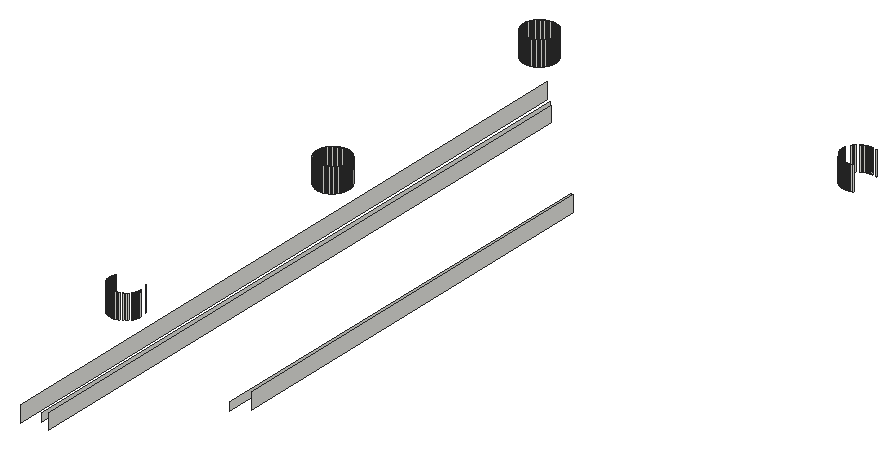
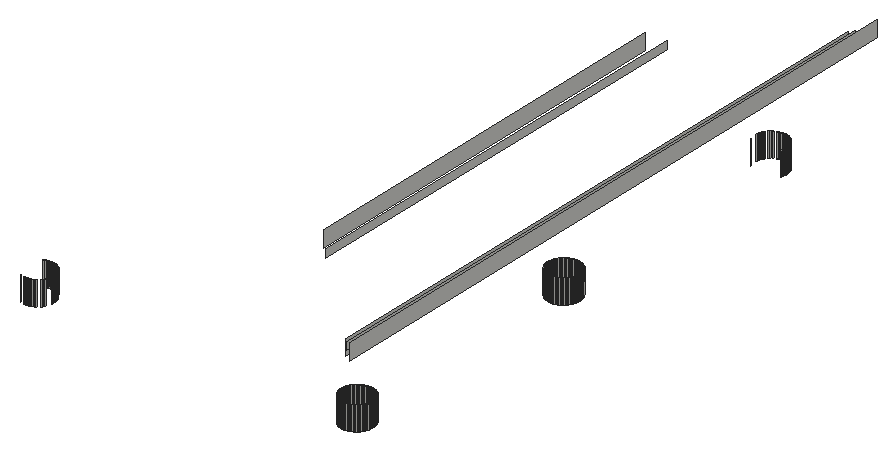
# SketchUp Ruby script. Lengths in millimetres.
U = 1.mm
M = Sketchup.active_model
def pt(a) = Geom::Point3d.new(a.map { |v| v * U })
def face(e, loops, mat)
  f = e.add_face(loops[0].map { |a| pt(a) })
  loops[1..].each { |l| e.add_face(l.map { |a| pt(a) }).erase! }
  f.material = f.back_material = mat if mat
  f
end
# faces: each face lists its corners as indices into pts; further lists are holes
def faces(e, pts, list, mat = nil) = list.each { |f| face(e, (f[0].is_a?(Array) ? f : [f]).map { |l| l.map { |i| pts[i] } }, mat) }
# xy, xz, yz: faces in a plane at the given z, y or x. An outline is a flat list of corners, or four numbers for a rectangle; further outlines are holes
def ring(l) = l.size == 4 ? [[l[0], l[1]], [l[2], l[1]], [l[2], l[3]], [l[0], l[3]]] : l.each_slice(2).to_a
def flat(e, list, mat, &to3) = list.each { |f| face(e, (f[0].is_a?(Array) ? f : [f]).map { |l| ring(l).map { |u, v| to3.(u, v) } }, mat) }
def xy(e, z, list, mat = nil) = flat(e, list, mat) { |x, y| [x, y, z] }
def xz(e, y, list, mat = nil) = flat(e, list, mat) { |x, z| [x, y, z] }
def yz(e, x, list, mat = nil) = flat(e, list, mat) { |y, z| [x, y, z] }
def lines(e, pts, list) = list.each { |a, b| e.add_line(pt(pts[a]), pt(pts[b])) }
# prism: a flat outline (further loops are holes) pulled along v
def prism(e, loops, v, mat = nil)
  f = face(e, loops, mat); d = Geom::Vector3d.new(v.map { |x| x * U })
  f.pushpull(f.normal.samedirection?(d) ? d.length : -d.length)
end
def box(e, o, s, mat = nil) = prism(e, [[o, [o[0] + s[0], o[1], o[2]], [o[0] + s[0], o[1] + s[1], o[2]], [o[0], o[1] + s[1], o[2]]]], [0, 0, s[2]], mat)
def at(x, y, z, deg = 0) = Geom::Transformation.translation(pt([x, y, z])) * Geom::Transformation.rotation(ORIGIN, Z_AXIS, deg.degrees)
def axes(o, x, y, z) = Geom::Transformation.new([*x, 0, *y, 0, *z, 0, *pt(o).to_a, 1])
def part(name) = M.definitions.add(name)
# library, detail: a bought-in or finely detailed component or shape, given as its bounding box
def library(name, o, s) = part(name).tap { |d| box(d.entities, o, s) }
def detail(e, o, s) = box(e.add_group.entities, o, s)
def put(e, d, t, mat = nil) = e.add_instance(d, t).tap { |i| i.material = mat if mat }
def group(e, t, mat = nil) = e.add_group.tap { |g| g.transformation = t; g.material = mat if mat }.entities
root = M.entities
yz(root,635,[[406.4,2743.2,2489.2,2794]])
yz(root,673.1,[[444.5,2743.2,2451.1,2766.6]])
yz(root,685.8,[[457.2,2718.2,2438.4,2766.6]])
yz(root,1003.3,[[774.7,2743.2,2120.9,2768.6]])
yz(root,1041.4,[[812.8,2743.2,2082.8,2794]])
p = [[454,995.6,2718.2],[454,995.6,2794],[457.2,995.5,2794],[457.2,995.5,2718.2],[460.4,995.6,2794],[460.4,995.6,2718.2],
  [450.8,995.9,2718.2],[450.8,995.9,2794],[463.6,995.9,2794],[463.6,995.9,2718.2],[447.7,996.4,2718.2],[447.7,996.4,2794],
  [466.7,996.4,2794],[466.7,996.4,2718.2],[444.6,997.1,2718.2],[444.6,997.1,2794],[469.8,997.1,2794],[469.8,997.1,2718.2],
  [441.5,998,2718.2],[441.5,998,2794],[472.9,998,2794],[472.9,998,2718.2],[438.5,999,2718.2],[438.5,999,2794],
  [475.9,999,2794],[475.9,999,2718.2],[435.6,1000.3,2718.2],[435.6,1000.3,2794],[432.7,1001.8,2718.2],[432.7,1001.8,2794],
  [481.7,1001.8,2718.2],[481.7,1001.8,2794],[484.4,1003.4,2794],[484.4,1003.4,2718.2],[424.8,1007.1,2718.2],[424.8,1007.1,2794],
  [427.3,1005.2,2794],[427.3,1005.2,2718.2],[489.6,1007.1,2718.2],[489.6,1007.1,2794],[492,1009.2,2794],[492,1009.2,2718.2],
  [494.2,1011.5,2794],[494.2,1011.5,2718.2],[418.1,1013.9,2718.2],[418.1,1013.9,2794],[420.2,1011.5,2794],[420.2,1011.5,2718.2],
  [498.3,1016.4,2718.2],[498.3,1016.4,2794],[500.1,1019,2794],[500.1,1019,2718.2],[412.7,1021.8,2718.2],[412.7,1021.8,2794],
  [414.3,1019,2794],[414.3,1019,2718.2],[501.7,1021.8,2794],[501.7,1021.8,2718.2],[411.2,1024.6,2718.2],[411.2,1024.6,2794],
  [503.2,1024.6,2794],[503.2,1024.6,2718.2],[410,1027.6,2718.2],[410,1027.6,2794],[504.4,1027.6,2794],[504.4,1027.6,2718.2],
  [408.9,1030.6,2718.2],[408.9,1030.6,2794],[505.5,1030.6,2794],[505.5,1030.6,2718.2],[408,1033.6,2718.2],[408,1033.6,2794],
  [506.4,1033.6,2794],[506.4,1033.6,2718.2],[507.1,1036.7,2794],[507.1,1036.7,2718.2],[507.6,1039.9,2794],[507.6,1039.9,2718.2],
  [406.5,1043.1,2718.2],[406.5,1043.1,2794],[406.8,1039.9,2794],[406.8,1039.9,2718.2],[507.9,1043.1,2794],[507.9,1043.1,2718.2],
  [406.4,1046.3,2718.2],[406.4,1046.3,2794],[406.5,1049.5,2718.2],[406.5,1049.5,2794],[406.8,1052.6,2718.2],[406.8,1052.6,2794],
  [407.3,1055.8,2718.2],[407.3,1055.8,2794],[408,1058.9,2718.2],[408,1058.9,2794],[408.9,1062,2718.2],[408.9,1062,2794],
  [410,1065,2718.2],[410,1065,2794],[504.4,1065,2718.2],[504.4,1065,2794],[503.2,1067.9,2794],[503.2,1067.9,2718.2],
  [501.7,1070.7,2794],[501.7,1070.7,2718.2],[454,1813.2,2718.2],[454,1813.2,2794],[457.2,1813.1,2794],[457.2,1813.1,2718.2],
  [460.4,1813.2,2794],[460.4,1813.2,2718.2],[450.8,1813.5,2718.2],[450.8,1813.5,2794],[463.6,1813.5,2794],[463.6,1813.5,2718.2],
  [447.7,1814,2718.2],[447.7,1814,2794],[466.7,1814,2794],[466.7,1814,2718.2],[444.6,1814.7,2718.2],[444.6,1814.7,2794],
  [469.8,1814.7,2794],[469.8,1814.7,2718.2],[441.5,1815.6,2718.2],[441.5,1815.6,2794],[472.9,1815.6,2794],[472.9,1815.6,2718.2],
  [438.5,1816.7,2718.2],[438.5,1816.7,2794],[475.9,1816.7,2794],[475.9,1816.7,2718.2],[435.6,1818,2718.2],[435.6,1818,2794],
  [478.8,1818,2794],[478.8,1818,2718.2],[432.7,1819.4,2718.2],[432.7,1819.4,2794],[481.7,1819.4,2794],[481.7,1819.4,2718.2],
  [430,1821,2718.2],[430,1821,2794],[484.4,1821,2794],[484.4,1821,2718.2],[427.3,1822.8,2718.2],[427.3,1822.8,2794],
  [487.1,1822.8,2794],[487.1,1822.8,2718.2],[424.8,1824.8,2718.2],[424.8,1824.8,2794],[489.6,1824.8,2794],[489.6,1824.8,2718.2],
  [422.4,1826.9,2718.2],[422.4,1826.9,2794],[492,1826.9,2794],[492,1826.9,2718.2],[420.2,1829.2,2718.2],[420.2,1829.2,2794],
  [494.2,1829.2,2794],[494.2,1829.2,2718.2],[418.1,1831.6,2718.2],[418.1,1831.6,2794],[496.3,1831.6,2794],[496.3,1831.6,2718.2],
  [416.1,1834.1,2718.2],[416.1,1834.1,2794],[498.3,1834.1,2794],[498.3,1834.1,2718.2],[414.3,1836.7,2718.2],[414.3,1836.7,2794],
  [500.1,1836.7,2794],[500.1,1836.7,2718.2],[412.7,1839.5,2718.2],[412.7,1839.5,2794],[501.7,1839.5,2794],[501.7,1839.5,2718.2],
  [411.2,1842.3,2718.2],[411.2,1842.3,2794],[503.2,1842.3,2794],[503.2,1842.3,2718.2],[410,1845.2,2718.2],[410,1845.2,2794],
  [504.4,1845.2,2794],[504.4,1845.2,2718.2],[408.9,1848.2,2718.2],[408.9,1848.2,2794],[505.5,1848.2,2794],[505.5,1848.2,2718.2],
  [408,1851.3,2718.2],[408,1851.3,2794],[506.4,1851.3,2794],[506.4,1851.3,2718.2],[407.3,1854.4,2718.2],[407.3,1854.4,2794],
  [507.1,1854.4,2794],[507.1,1854.4,2718.2],[406.8,1857.6,2718.2],[406.8,1857.6,2794],[507.6,1857.6,2794],[507.6,1857.6,2718.2],
  [406.5,1860.7,2718.2],[406.5,1860.7,2794],[507.9,1860.7,2794],[507.9,1860.7,2718.2],[406.4,1863.9,2718.2],[406.4,1863.9,2794],
  [508,1863.9,2794],[508,1863.9,2718.2],[406.5,1867.1,2718.2],[406.5,1867.1,2794],[507.9,1867.1,2794],[507.9,1867.1,2718.2],
  [406.8,1870.3,2718.2],[406.8,1870.3,2794],[507.6,1870.3,2794],[507.6,1870.3,2718.2],[407.3,1873.5,2718.2],[407.3,1873.5,2794],
  [507.1,1873.5,2794],[507.1,1873.5,2718.2],[408,1876.6,2718.2],[408,1876.6,2794],[506.4,1876.6,2794],[506.4,1876.6,2718.2],
  [408.9,1879.6,2718.2],[408.9,1879.6,2794],[505.5,1879.6,2794],[505.5,1879.6,2718.2],[410,1882.6,2718.2],[410,1882.6,2794],
  [504.4,1882.6,2794],[504.4,1882.6,2718.2],[411.2,1885.6,2718.2],[411.2,1885.6,2794],[503.2,1885.6,2794],[503.2,1885.6,2718.2],
  [412.7,1888.4,2718.2],[412.7,1888.4,2794],[501.7,1888.4,2794],[501.7,1888.4,2718.2],[414.3,1891.2,2718.2],[414.3,1891.2,2794],
  [500.1,1891.2,2794],[500.1,1891.2,2718.2],[416.1,1893.8,2718.2],[416.1,1893.8,2794],[498.3,1893.8,2794],[498.3,1893.8,2718.2],
  [418.1,1896.3,2718.2],[418.1,1896.3,2794],[496.3,1896.3,2794],[496.3,1896.3,2718.2],[420.2,1898.7,2718.2],[420.2,1898.7,2794],
  [494.2,1898.7,2794],[494.2,1898.7,2718.2],[422.4,1901,2718.2],[422.4,1901,2794],[492,1901,2794],[492,1901,2718.2],
  [424.8,1903.1,2718.2],[424.8,1903.1,2794],[489.6,1903.1,2794],[489.6,1903.1,2718.2],[427.3,1905,2718.2],[427.3,1905,2794],
  [487.1,1905,2794],[487.1,1905,2718.2],[430,1906.8,2718.2],[430,1906.8,2794],[484.4,1906.8,2794],[484.4,1906.8,2718.2],
  [432.7,1908.4,2718.2],[432.7,1908.4,2794],[481.7,1908.4,2794],[481.7,1908.4,2718.2],[435.6,1909.9,2718.2],[435.6,1909.9,2794],
  [478.8,1909.9,2794],[478.8,1909.9,2718.2],[438.5,1911.2,2718.2],[438.5,1911.2,2794],[475.9,1911.2,2794],[475.9,1911.2,2718.2],
  [441.5,1912.2,2718.2],[441.5,1912.2,2794],[472.9,1912.2,2794],[472.9,1912.2,2718.2],[444.6,1913.1,2718.2],[444.6,1913.1,2794],
  [469.8,1913.1,2794],[469.8,1913.1,2718.2],[447.7,1913.8,2718.2],[447.7,1913.8,2794],[466.7,1913.8,2794],[466.7,1913.8,2718.2],
  [450.8,1914.3,2718.2],[450.8,1914.3,2794],[463.6,1914.3,2794],[463.6,1914.3,2718.2],[454,1914.6,2718.2],[454,1914.6,2794],
  [460.4,1914.6,2794],[460.4,1914.6,2718.2],[457.2,1914.7,2718.2],[457.2,1914.7,2794],[454,2630.9,2718.2],[454,2630.9,2794],
  [457.2,2630.8,2794],[457.2,2630.8,2718.2],[460.4,2630.9,2794],[460.4,2630.9,2718.2],[1465.5,2630.8,2794],[1465.5,2630.8,2718.2],
  [1462.3,2630.9,2718.2],[1462.3,2630.9,2794],[1468.7,2630.9,2794],[1468.7,2630.9,2718.2],[450.8,2631.2,2718.2],[450.8,2631.2,2794],
  [463.6,2631.2,2794],[463.6,2631.2,2718.2],[1459.2,2631.2,2718.2],[1459.2,2631.2,2794],[1471.9,2631.2,2794],[1471.9,2631.2,2718.2],
  [447.7,2631.7,2718.2],[447.7,2631.7,2794],[466.7,2631.7,2794],[466.7,2631.7,2718.2],[1456,2631.7,2718.2],[1456,2631.7,2794],
  [1475.1,2631.7,2794],[1475.1,2631.7,2718.2],[444.6,2632.4,2718.2],[444.6,2632.4,2794],[469.8,2632.4,2794],[469.8,2632.4,2718.2],
  [1452.9,2632.4,2718.2],[1452.9,2632.4,2794],[1478.2,2632.4,2794],[1478.2,2632.4,2718.2],[441.5,2633.3,2718.2],[441.5,2633.3,2794],
  [472.9,2633.3,2794],[472.9,2633.3,2718.2],[1449.8,2633.3,2718.2],[1449.8,2633.3,2794],[1481.2,2633.3,2794],[1481.2,2633.3,2718.2],
  [438.5,2634.4,2718.2],[438.5,2634.4,2794],[475.9,2634.4,2794],[475.9,2634.4,2718.2],[1446.8,2634.4,2718.2],[1446.8,2634.4,2794],
  [1484.2,2634.4,2794],[1484.2,2634.4,2718.2],[435.6,2635.6,2718.2],[435.6,2635.6,2794],[478.8,2635.6,2794],[478.8,2635.6,2718.2],
  [1443.9,2635.6,2718.2],[1443.9,2635.6,2794],[1487.2,2635.6,2794],[1487.2,2635.6,2718.2],[432.7,2637.1,2718.2],[432.7,2637.1,2794],
  [481.7,2637.1,2794],[481.7,2637.1,2718.2],[1441.1,2637.1,2718.2],[1441.1,2637.1,2794],[430,2638.7,2718.2],[430,2638.7,2794],
  [484.4,2638.7,2794],[484.4,2638.7,2718.2],[1438.3,2638.7,2718.2],[1438.3,2638.7,2794],[427.3,2640.5,2718.2],[427.3,2640.5,2794],
  [487.1,2640.5,2794],[487.1,2640.5,2718.2],[1435.7,2640.5,2718.2],[1435.7,2640.5,2794],[424.8,2642.5,2718.2],[424.8,2642.5,2794],
  [489.6,2642.5,2794],[489.6,2642.5,2718.2],[1433.2,2642.5,2718.2],[1433.2,2642.5,2794],[422.4,2644.6,2718.2],[422.4,2644.6,2794],
  [492,2644.6,2794],[492,2644.6,2718.2],[1430.8,2644.6,2718.2],[1430.8,2644.6,2794],[420.2,2646.8,2718.2],[420.2,2646.8,2794],
  [494.2,2646.8,2794],[494.2,2646.8,2718.2],[418.1,2649.2,2718.2],[418.1,2649.2,2794],[496.3,2649.2,2794],[496.3,2649.2,2718.2],
  [416.1,2651.7,2718.2],[416.1,2651.7,2794],[498.3,2651.7,2794],[498.3,2651.7,2718.2],[414.3,2654.4,2718.2],[414.3,2654.4,2794],
  [500.1,2654.4,2794],[500.1,2654.4,2718.2],[412.7,2657.1,2718.2],[412.7,2657.1,2794],[501.7,2657.1,2794],[501.7,2657.1,2718.2],
  [411.2,2660,2718.2],[411.2,2660,2794],[503.2,2660,2794],[503.2,2660,2718.2],[410,2662.9,2718.2],[410,2662.9,2794],
  [504.4,2662.9,2794],[504.4,2662.9,2718.2],[1419.6,2660,2794],[1419.6,2660,2718.2],[1418.3,2662.9,2718.2],[1418.3,2662.9,2794],
  [408.9,2665.9,2718.2],[408.9,2665.9,2794],[505.5,2665.9,2794],[505.5,2665.9,2718.2],[408,2669,2718.2],[408,2669,2794],
  [506.4,2669,2794],[506.4,2669,2718.2],[407.3,2672.1,2718.2],[407.3,2672.1,2794],[507.1,2672.1,2794],[507.1,2672.1,2718.2],
  [1416.3,2669,2794],[1416.3,2669,2718.2],[1415.6,2672.1,2718.2],[1415.6,2672.1,2794],[406.8,2675.2,2718.2],[406.8,2675.2,2794],
  [507.6,2675.2,2794],[507.6,2675.2,2718.2],[1415.1,2675.2,2718.2],[1415.1,2675.2,2794],[406.5,2678.4,2718.2],[406.5,2678.4,2794],
  [507.9,2678.4,2794],[507.9,2678.4,2718.2],[1414.8,2678.4,2718.2],[1414.8,2678.4,2794],[406.4,2681.6,2718.2],[406.4,2681.6,2794],
  [508,2681.6,2794],[508,2681.6,2718.2],[1414.7,2681.6,2718.2],[1414.7,2681.6,2794],[406.5,2684.8,2718.2],[406.5,2684.8,2794],
  [507.9,2684.8,2794],[507.9,2684.8,2718.2],[1414.8,2684.8,2718.2],[1414.8,2684.8,2794],[406.8,2688,2718.2],[406.8,2688,2794],
  [507.6,2688,2794],[507.6,2688,2718.2],[1415.1,2688,2718.2],[1415.1,2688,2794],[407.3,2691.1,2718.2],[407.3,2691.1,2794],
  [507.1,2691.1,2794],[507.1,2691.1,2718.2],[1415.6,2691.1,2718.2],[1415.6,2691.1,2794],[408,2694.2,2718.2],[408,2694.2,2794],
  [506.4,2694.2,2794],[506.4,2694.2,2718.2],[408.9,2697.3,2718.2],[408.9,2697.3,2794],[505.5,2697.3,2794],[505.5,2697.3,2718.2],
  [410,2700.3,2718.2],[410,2700.3,2794],[504.4,2700.3,2794],[504.4,2700.3,2718.2],[411.2,2703.2,2718.2],[411.2,2703.2,2794],
  [503.2,2703.2,2794],[503.2,2703.2,2718.2],[412.7,2706.1,2718.2],[412.7,2706.1,2794],[501.7,2706.1,2794],[501.7,2706.1,2718.2],
  [414.3,2708.8,2718.2],[414.3,2708.8,2794],[500.1,2708.8,2794],[500.1,2708.8,2718.2],[1421,2706.1,2794],[1421,2706.1,2718.2],
  [1422.6,2708.8,2718.2],[1422.6,2708.8,2794],[416.1,2711.5,2718.2],[416.1,2711.5,2794],[498.3,2711.5,2794],[498.3,2711.5,2718.2],
  [1424.4,2711.5,2718.2],[1424.4,2711.5,2794],[418.1,2714,2718.2],[418.1,2714,2794],[496.3,2714,2794],[496.3,2714,2718.2],
  [1426.4,2714,2718.2],[1426.4,2714,2794],[420.2,2716.4,2718.2],[420.2,2716.4,2794],[494.2,2716.4,2794],[494.2,2716.4,2718.2],
  [1428.5,2716.4,2718.2],[1428.5,2716.4,2794],[422.4,2718.6,2718.2],[422.4,2718.6,2794],[492,2718.6,2794],[492,2718.6,2718.2],
  [424.8,2720.7,2718.2],[424.8,2720.7,2794],[489.6,2720.7,2794],[489.6,2720.7,2718.2],[427.3,2722.7,2718.2],[427.3,2722.7,2794],
  [487.1,2722.7,2794],[487.1,2722.7,2718.2],[430,2724.5,2718.2],[430,2724.5,2794],[484.4,2724.5,2794],[484.4,2724.5,2718.2],
  [1435.7,2722.7,2794],[1435.7,2722.7,2718.2],[1438.3,2724.5,2718.2],[1438.3,2724.5,2794],[432.7,2726.1,2718.2],[432.7,2726.1,2794],
  [481.7,2726.1,2794],[481.7,2726.1,2718.2],[1441.1,2726.1,2718.2],[1441.1,2726.1,2794],[435.6,2727.6,2718.2],[435.6,2727.6,2794],
  [478.8,2727.6,2794],[478.8,2727.6,2718.2],[1443.9,2727.6,2718.2],[1443.9,2727.6,2794],[438.5,2728.8,2718.2],[438.5,2728.8,2794],
  [475.9,2728.8,2794],[475.9,2728.8,2718.2],[1446.8,2728.8,2718.2],[1446.8,2728.8,2794],[441.5,2729.9,2718.2],[441.5,2729.9,2794],
  [472.9,2729.9,2794],[472.9,2729.9,2718.2],[1449.8,2729.9,2718.2],[1449.8,2729.9,2794],[1481.2,2729.9,2794],[1481.2,2729.9,2718.2],
  [1484.2,2728.8,2718.2],[1484.2,2728.8,2794],[444.6,2730.8,2718.2],[444.6,2730.8,2794],[469.8,2730.8,2794],[469.8,2730.8,2718.2],
  [1452.9,2730.8,2718.2],[1452.9,2730.8,2794],[447.7,2731.5,2718.2],[447.7,2731.5,2794],[466.7,2731.5,2794],[466.7,2731.5,2718.2],
  [1456,2731.5,2718.2],[1456,2731.5,2794],[450.8,2732,2718.2],[450.8,2732,2794],[463.6,2732,2794],[463.6,2732,2718.2],
  [1459.2,2732,2718.2],[1459.2,2732,2794],[454,2732.3,2718.2],[454,2732.3,2794],[460.4,2732.3,2794],[460.4,2732.3,2718.2],
  [1462.3,2732.3,2718.2],[1462.3,2732.3,2794],[1468.7,2732.3,2794],[1468.7,2732.3,2718.2],[1471.9,2732,2718.2],[1471.9,2732,2794],
  [457.2,2732.4,2718.2],[457.2,2732.4,2794],[1465.5,2732.4,2718.2],[1465.5,2732.4,2794]]
faces(root,p,[[0,1,2,3],[3,2,4,5],[6,7,1,0],[5,4,8,9],[10,11,7,6],[9,8,12,13],[14,15,11,10],[13,12,16,17],
  [18,19,15,14],[17,16,20,21],[22,23,19,18],[21,20,24,25],[26,27,23,22],[28,29,27,26],[30,31,32,33],[34,35,36,37],
  [38,39,40,41],[41,40,42,43],[44,45,46,47],[48,49,50,51],[52,53,54,55],[51,50,56,57],[58,59,53,52],[57,56,60,61],
  [62,63,59,58],[61,60,64,65],[66,67,63,62],[65,64,68,69],[70,71,67,66],[69,68,72,73],[73,72,74,75],[75,74,76,77],
  [78,79,80,81],[77,76,82,83],[84,85,79,78],[86,87,85,84],[88,89,87,86],[90,91,89,88],[92,93,91,90],[94,95,93,92],
  [96,97,95,94],[98,99,100,101],[101,100,102,103],[104,105,106,107],[107,106,108,109],[110,111,105,104],[109,108,112,113],[114,115,111,110],
  [113,112,116,117],[118,119,115,114],[117,116,120,121],[122,123,119,118],[121,120,124,125],[126,127,123,122],[125,124,128,129],[130,131,127,126],
  [129,128,132,133],[134,135,131,130],[133,132,136,137],[138,139,135,134],[137,136,140,141],[142,143,139,138],[141,140,144,145],[146,147,143,142],
  [145,144,148,149],[150,151,147,146],[149,148,152,153],[154,155,151,150],[153,152,156,157],[158,159,155,154],[157,156,160,161],[162,163,159,158],
  [161,160,164,165],[166,167,163,162],[165,164,168,169],[170,171,167,166],[169,168,172,173],[174,175,171,170],[173,172,176,177],[178,179,175,174],
  [177,176,180,181],[182,183,179,178],[181,180,184,185],[186,187,183,182],[185,184,188,189],[190,191,187,186],[189,188,192,193],[194,195,191,190],
  [193,192,196,197],[198,199,195,194],[197,196,200,201],[202,203,199,198],[201,200,204,205],[206,207,203,202],[205,204,208,209],[210,211,207,206],
  [209,208,212,213],[214,215,211,210],[213,212,216,217],[218,219,215,214],[217,216,220,221],[222,223,219,218],[221,220,224,225],[226,227,223,222],
  [225,224,228,229],[230,231,227,226],[229,228,232,233],[234,235,231,230],[233,232,236,237],[238,239,235,234],[237,236,240,241],[242,243,239,238],
  [241,240,244,245],[246,247,243,242],[245,244,248,249],[250,251,247,246],[249,248,252,253],[254,255,251,250],[253,252,256,257],[258,259,255,254],
  [257,256,260,261],[262,263,259,258],[261,260,264,265],[266,267,263,262],[265,264,268,269],[270,271,267,266],[269,268,272,273],[274,275,271,270],
  [273,272,276,277],[278,279,275,274],[277,276,280,281],[282,283,279,278],[281,280,284,285],[286,287,283,282],[285,284,288,289],[290,291,287,286],
  [289,288,292,293],[294,295,291,290],[293,292,296,297],[298,299,295,294],[297,296,300,301],[302,303,299,298],[301,300,303,302],[304,305,306,307],
  [307,306,308,309],[310,311,312,313],[314,315,311,310],[316,317,305,304],[309,308,318,319],[313,312,320,321],[322,323,315,314],[324,325,317,316],
  [319,318,326,327],[321,320,328,329],[330,331,323,322],[332,333,325,324],[327,326,334,335],[329,328,336,337],[338,339,331,330],[340,341,333,332],
  [335,334,342,343],[337,336,344,345],[346,347,339,338],[348,349,341,340],[343,342,350,351],[345,344,352,353],[354,355,347,346],[356,357,349,348],
  [351,350,358,359],[353,352,360,361],[362,363,355,354],[364,365,357,356],[359,358,366,367],[361,360,368,369],[370,371,365,364],[367,366,372,373],
  [369,368,374,375],[376,377,371,370],[373,372,378,379],[375,374,380,381],[382,383,377,376],[379,378,384,385],[381,380,386,387],[388,389,383,382],
  [385,384,390,391],[387,386,392,393],[394,395,389,388],[391,390,396,397],[398,399,395,394],[397,396,400,401],[402,403,399,398],[401,400,404,405],
  [406,407,403,402],[405,404,408,409],[410,411,407,406],[409,408,412,413],[414,415,411,410],[413,412,416,417],[418,419,415,414],[417,416,420,421],
  [422,423,424,425],[426,427,419,418],[421,420,428,429],[430,431,427,426],[429,428,432,433],[434,435,431,430],[433,432,436,437],[438,439,440,441],
  [442,443,435,434],[437,436,444,445],[441,440,446,447],[448,449,443,442],[445,444,450,451],[447,446,452,453],[454,455,449,448],[451,450,456,457],
  [453,452,458,459],[460,461,455,454],[457,456,462,463],[459,458,464,465],[466,467,461,460],[463,462,468,469],[465,464,470,471],[472,473,467,466],
  [469,468,474,475],[471,470,476,477],[478,479,473,472],[475,474,480,481],[482,483,479,478],[481,480,484,485],[486,487,483,482],[485,484,488,489],
  [490,491,487,486],[489,488,492,493],[494,495,491,490],[493,492,496,497],[498,499,495,494],[497,496,500,501],[502,503,504,505],[506,507,499,498],
  [501,500,508,509],[505,504,510,511],[512,513,507,506],[509,508,514,515],[511,510,516,517],[518,519,513,512],[515,514,520,521],[517,516,522,523],
  [524,525,519,518],[521,520,526,527],[528,529,525,524],[527,526,530,531],[532,533,529,528],[531,530,534,535],[536,537,533,532],[535,534,538,539],
  [540,541,542,543],[544,545,537,536],[539,538,546,547],[543,542,548,549],[550,551,545,544],[547,546,552,553],[549,548,554,555],[556,557,551,550],
  [553,552,558,559],[555,554,560,561],[562,563,557,556],[559,558,564,565],[561,560,566,567],[568,569,570,571],[572,573,563,562],[565,564,574,575],
  [567,566,576,577],[578,579,573,572],[575,574,580,581],[577,576,582,583],[584,585,579,578],[581,580,586,587],[583,582,588,589],[590,591,585,584],
  [587,586,592,593],[589,588,594,595],[596,597,598,599],[600,601,591,590],[593,592,601,600],[595,594,602,603],[603,602,597,596]])
